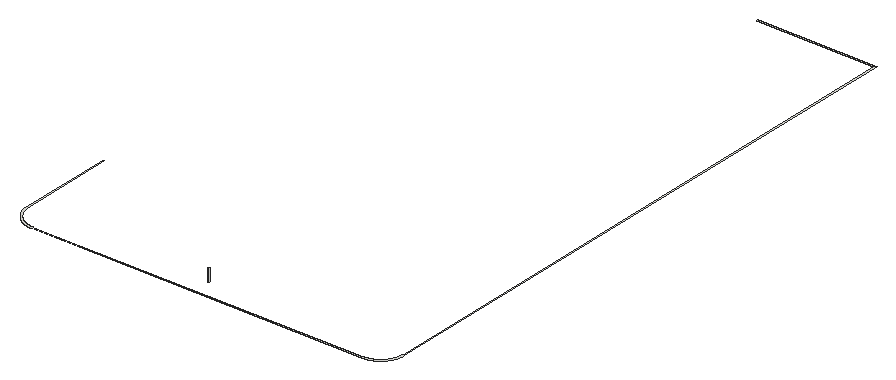
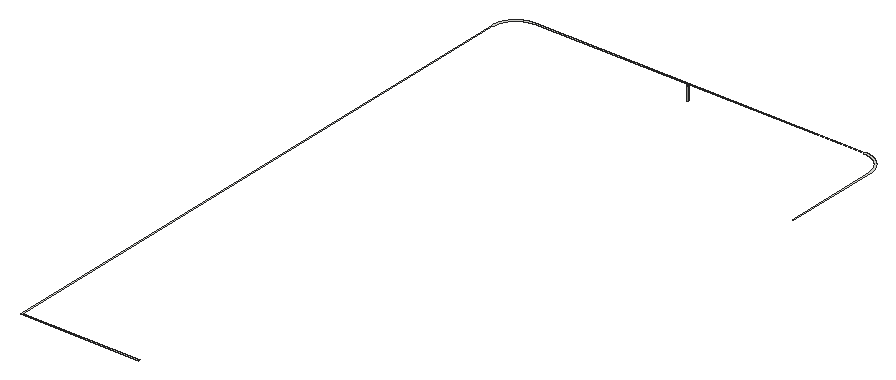
# SketchUp Ruby script. Lengths in inches.
U = 1.inch
M = Sketchup.active_model
def pt(a) = Geom::Point3d.new(a.map { |v| v * U })
def face(e, loops, mat)
  f = e.add_face(loops[0].map { |a| pt(a) })
  loops[1..].each { |l| e.add_face(l.map { |a| pt(a) }).erase! }
  f.material = f.back_material = mat if mat
  f
end
# faces: each face lists its corners as indices into pts; further lists are holes
def faces(e, pts, list, mat = nil) = list.each { |f| face(e, (f[0].is_a?(Array) ? f : [f]).map { |l| l.map { |i| pts[i] } }, mat) }
# xy, xz, yz: faces in a plane at the given z, y or x. An outline is a flat list of corners, or four numbers for a rectangle; further outlines are holes
def ring(l) = l.size == 4 ? [[l[0], l[1]], [l[2], l[1]], [l[2], l[3]], [l[0], l[3]]] : l.each_slice(2).to_a
def flat(e, list, mat, &to3) = list.each { |f| face(e, (f[0].is_a?(Array) ? f : [f]).map { |l| ring(l).map { |u, v| to3.(u, v) } }, mat) }
def xy(e, z, list, mat = nil) = flat(e, list, mat) { |x, y| [x, y, z] }
def xz(e, y, list, mat = nil) = flat(e, list, mat) { |x, z| [x, y, z] }
def yz(e, x, list, mat = nil) = flat(e, list, mat) { |y, z| [x, y, z] }
def lines(e, pts, list) = list.each { |a, b| e.add_line(pt(pts[a]), pt(pts[b])) }
# prism: a flat outline (further loops are holes) pulled along v
def prism(e, loops, v, mat = nil)
  f = face(e, loops, mat); d = Geom::Vector3d.new(v.map { |x| x * U })
  f.pushpull(f.normal.samedirection?(d) ? d.length : -d.length)
end
def box(e, o, s, mat = nil) = prism(e, [[o, [o[0] + s[0], o[1], o[2]], [o[0] + s[0], o[1] + s[1], o[2]], [o[0], o[1] + s[1], o[2]]]], [0, 0, s[2]], mat)
def at(x, y, z, deg = 0) = Geom::Transformation.translation(pt([x, y, z])) * Geom::Transformation.rotation(ORIGIN, Z_AXIS, deg.degrees)
def axes(o, x, y, z) = Geom::Transformation.new([*x, 0, *y, 0, *z, 0, *pt(o).to_a, 1])
def part(name) = M.definitions.add(name)
# library, detail: a bought-in or finely detailed component or shape, given as its bounding box
def library(name, o, s) = part(name).tap { |d| box(d.entities, o, s) }
def detail(e, o, s) = box(e.add_group.entities, o, s)
def put(e, d, t, mat = nil) = e.add_instance(d, t).tap { |i| i.material = mat if mat }
def group(e, t, mat = nil) = e.add_group.tap { |g| g.transformation = t; g.material = mat if mat }.entities
root = M.entities
xy(root,348.5,[[38.78,217,38.55,217.01,38.33,217.01,38.11,217.02,37.89,217.04,37.67,217.05,37.44,217.07,37.22,217.09,36.78,217.15,36.5625,217.18,36.34,217.21,36.12,217.25,35.9,217.28,35.68,217.33,35.47,217.37,35.03,217.47,34.82,217.52,34.6,217.58,34.39,217.64,34.17,217.7,33.96,217.76,33.54,217.9,33.33,217.98,33.12,218.05,32.49,218.29,32.09,218.47,31.88,218.5625,31.68,218.66,31.48,218.75,31.28,218.85,31.08,218.96,30.89,219.06,30.69,219.17,30.31,219.39,30.12,219.51,29.93,219.62,29.74,219.74,29.56,219.87,29.37,219.99,29.1875,220.12,29.01,220.25,28.65,220.51,28.48,220.65,28.3,220.79,27.96,221.07,27.79,221.22,27.46,221.52,27.14,221.82,26.82,222.14,26.52,222.46,26.22,222.79,26.07,222.96,25.79,223.3,25.65,223.48,25.51,223.65,25.25,224.01,25.12,224.1875,24.99,224.37,24.87,224.56,24.74,224.74,24.62,224.93,24.51,225.12,24.39,225.31,24.17,225.69,24.06,225.89,23.96,226.08,23.85,226.28,23.75,226.48,23.66,226.68,23.5625,226.88,23.47,227.09,23.29,227.49,23.05,228.12,22.98,228.33,22.9,228.54,22.76,228.96,22.7,229.17,22.64,229.39,22.58,229.6,22.52,229.82,22.47,230.03,22.37,230.47,22.33,230.68,22.28,230.9,22.25,231.12,22.21,231.34,22.18,231.5625,22.15,231.78,22.09,232.22,22.07,232.44,22.05,232.67,22.04,232.89,22.02,233.11,22.01,233.33,22.01,233.55,22,233.78,22,300,23,300,23,233.79,23.01,233.58,23.01,233.37,23.03,232.95,23.05,232.74,23.07,232.54,23.11,232.12,23.17,231.7,23.2,231.5,23.23,231.29,23.27,231.08,23.31,230.88,23.35,230.67,23.39,230.47,23.44,230.26,23.49,230.0625,23.55,229.86,23.6,229.66,23.78,229.06,23.99,228.46,24.0625,228.27,24.14,228.07,24.22,227.88,24.3,227.68,24.38,227.49,24.65,226.92,24.74,226.74,24.84,226.55,24.9375,226.37,25.04,226.18,25.14,226,25.47,225.46,25.58,225.29,25.7,225.11,25.8125,224.9375,25.93,224.77,26.06,224.6,26.18,224.43,26.31,224.26,26.43,224.09,26.57,223.93,26.83,223.61,27.11,223.29,27.39,222.99,27.54,222.84,27.6875,222.6875,27.84,222.54,27.99,222.39,28.29,222.11,28.61,221.83,28.93,221.57,29.09,221.43,29.26,221.31,29.43,221.18,29.6,221.06,29.77,220.93,29.9375,220.8125,30.11,220.7,30.29,220.58,30.46,220.47,31,220.14,31.18,220.04,31.37,219.9375,31.55,219.84,31.74,219.74,31.92,219.65,32.49,219.38,32.68,219.3,32.88,219.22,33.07,219.14,33.27,219.0625,33.46,218.99,34.06,218.78,34.66,218.6,34.86,218.55,35.0625,218.49,35.26,218.44,35.47,218.39,35.67,218.35,35.88,218.31,36.08,218.27,36.29,218.23,36.5,218.2,36.7,218.17,37.12,218.11,37.54,218.07,37.74,218.05,37.95,218.03,38.37,218.01,38.58,218.01,38.79,218,270.21,218,270.42,218.01,270.63,218.01,271.05,218.03,271.26,218.05,271.46,218.07,271.88,218.11,272.3,218.17,272.5,218.2,272.71,218.23,272.92,218.27,273.12,218.31,273.33,218.35,273.53,218.39,273.74,218.44,273.9375,218.49,274.14,218.55,274.34,218.6,274.94,218.78,275.54,218.99,275.73,219.0625,275.93,219.14,276.12,219.22,276.32,219.3,276.51,219.38,277.08,219.65,277.26,219.74,277.45,219.84,277.63,219.9375,277.82,220.04,278,220.14,278.54,220.47,278.71,220.58,278.89,220.7,279.0625,220.8125,279.23,220.93,279.4,221.06,279.57,221.18,279.74,221.31,279.91,221.43,280.07,221.57,280.39,221.83,280.71,222.11,281.01,222.39,281.16,222.54,281.3125,222.6875,281.46,222.84,281.61,222.99,281.89,223.29,282.17,223.61,282.43,223.93,282.57,224.09,282.69,224.26,282.82,224.43,282.94,224.6,283.07,224.77,283.1875,224.9375,283.3,225.11,283.42,225.29,283.53,225.46,283.86,226,283.96,226.18,284.0625,226.37,284.16,226.55,284.26,226.74,284.35,226.92,284.62,227.49,284.7,227.68,284.78,227.88,284.86,228.07,284.9375,228.27,285.01,228.46,285.22,229.06,285.4,229.66,285.45,229.86,285.51,230.0625,285.56,230.26,285.61,230.47,285.65,230.67,285.69,230.88,285.73,231.08,285.77,231.29,285.8,231.5,285.83,231.7,285.89,232.12,285.93,232.54,285.95,232.74,285.97,232.95,285.99,233.37,285.99,233.58,286,233.79,286,646,204,646,204,647,287,647,287,233.78,286.99,233.55,286.99,233.33,286.98,233.11,286.96,232.89,286.95,232.67,286.93,232.44,286.91,232.22,286.85,231.78,286.82,231.5625,286.79,231.34,286.75,231.12,286.72,230.9,286.67,230.68,286.63,230.47,286.53,230.03,286.48,229.82,286.42,229.6,286.36,229.39,286.3,229.17,286.24,228.96,286.1,228.54,286.02,228.33,285.95,228.12,285.71,227.49,285.53,227.09,285.4375,226.88,285.34,226.68,285.25,226.48,285.15,226.28,285.04,226.08,284.94,225.89,284.83,225.69,284.61,225.31,284.49,225.12,284.38,224.93,284.26,224.74,284.13,224.56,284.01,224.37,283.88,224.1875,283.75,224.01,283.49,223.65,283.35,223.48,283.21,223.3,282.93,222.96,282.78,222.79,282.48,222.46,282.18,222.14,281.86,221.82,281.54,221.52,281.21,221.22,281.04,221.07,280.7,220.79,280.52,220.65,280.35,220.51,279.99,220.25,279.8125,220.12,279.63,219.99,279.44,219.87,279.26,219.74,279.07,219.62,278.88,219.51,278.69,219.39,278.31,219.17,278.11,219.06,277.92,218.96,277.72,218.85,277.52,218.75,277.32,218.66,277.12,218.5625,276.91,218.47,276.51,218.29,275.88,218.05,275.67,217.98,275.46,217.9,275.04,217.76,274.83,217.7,274.61,217.64,274.4,217.58,274.18,217.52,273.97,217.47,273.53,217.37,273.32,217.33,273.1,217.28,272.88,217.25,272.66,217.21,272.4375,217.18,272.22,217.15,271.78,217.09,271.56,217.07,271.33,217.05,271.11,217.04,270.89,217.02,270.67,217.01,270.45,217.01,270.22,217]])
p = [[151.12,231.11,357],[151.58,231.4375,357],[151.58,231.4375,348],[151.12,231.11,348],[152.03,231.78,357],[152.03,231.78,348]]
faces(root,p,[[0,1,2,3],[1,4,5,2]])
